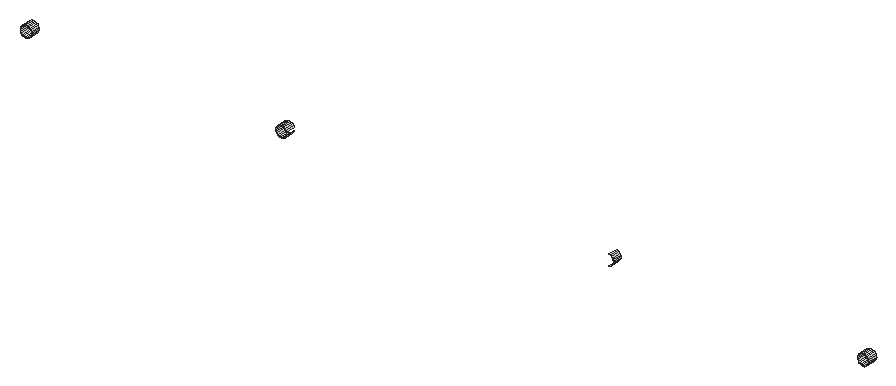
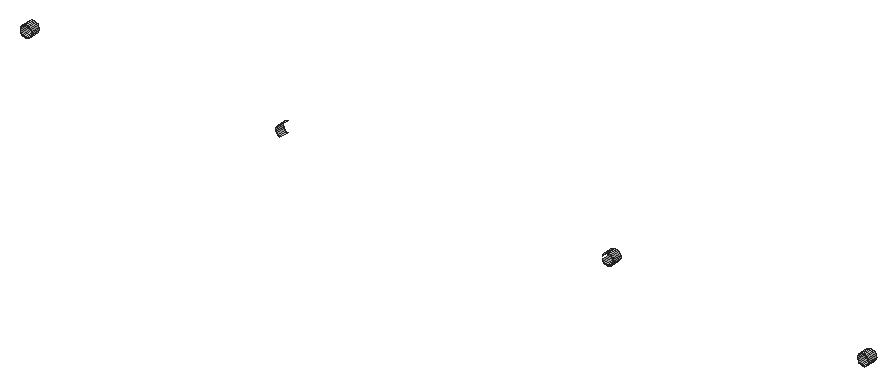
# SketchUp Ruby script. Lengths in inches.
U = 1.inch
M = Sketchup.active_model
def pt(a) = Geom::Point3d.new(a.map { |v| v * U })
def face(e, loops, mat)
  f = e.add_face(loops[0].map { |a| pt(a) })
  loops[1..].each { |l| e.add_face(l.map { |a| pt(a) }).erase! }
  f.material = f.back_material = mat if mat
  f
end
# faces: each face lists its corners as indices into pts; further lists are holes
def faces(e, pts, list, mat = nil) = list.each { |f| face(e, (f[0].is_a?(Array) ? f : [f]).map { |l| l.map { |i| pts[i] } }, mat) }
# xy, xz, yz: faces in a plane at the given z, y or x. An outline is a flat list of corners, or four numbers for a rectangle; further outlines are holes
def ring(l) = l.size == 4 ? [[l[0], l[1]], [l[2], l[1]], [l[2], l[3]], [l[0], l[3]]] : l.each_slice(2).to_a
def flat(e, list, mat, &to3) = list.each { |f| face(e, (f[0].is_a?(Array) ? f : [f]).map { |l| ring(l).map { |u, v| to3.(u, v) } }, mat) }
def xy(e, z, list, mat = nil) = flat(e, list, mat) { |x, y| [x, y, z] }
def xz(e, y, list, mat = nil) = flat(e, list, mat) { |x, z| [x, y, z] }
def yz(e, x, list, mat = nil) = flat(e, list, mat) { |y, z| [x, y, z] }
def lines(e, pts, list) = list.each { |a, b| e.add_line(pt(pts[a]), pt(pts[b])) }
# prism: a flat outline (further loops are holes) pulled along v
def prism(e, loops, v, mat = nil)
  f = face(e, loops, mat); d = Geom::Vector3d.new(v.map { |x| x * U })
  f.pushpull(f.normal.samedirection?(d) ? d.length : -d.length)
end
def box(e, o, s, mat = nil) = prism(e, [[o, [o[0] + s[0], o[1], o[2]], [o[0] + s[0], o[1] + s[1], o[2]], [o[0], o[1] + s[1], o[2]]]], [0, 0, s[2]], mat)
def at(x, y, z, deg = 0) = Geom::Transformation.translation(pt([x, y, z])) * Geom::Transformation.rotation(ORIGIN, Z_AXIS, deg.degrees)
def axes(o, x, y, z) = Geom::Transformation.new([*x, 0, *y, 0, *z, 0, *pt(o).to_a, 1])
def part(name) = M.definitions.add(name)
# library, detail: a bought-in or finely detailed component or shape, given as its bounding box
def library(name, o, s) = part(name).tap { |d| box(d.entities, o, s) }
def detail(e, o, s) = box(e.add_group.entities, o, s)
def put(e, d, t, mat = nil) = e.add_instance(d, t).tap { |i| i.material = mat if mat }
def group(e, t, mat = nil) = e.add_group.tap { |g| g.transformation = t; g.material = mat if mat }.entities
root = M.entities
p = [[2670.92,801.78,132.03],[2671.19,801.78,131.92],[2671.19,799.91,131.92],[2670.92,799.91,132.03],[2671.48,801.78,131.88],[2671.48,799.91,131.88],
  [2671.78,801.78,131.92],[2671.78,799.91,131.92],[2672.05,801.78,132.03],[2672.05,799.91,132.03],[2722.05,801.78,132.03],[2722.32,801.78,131.92],
  [2722.32,799.91,131.92],[2722.05,799.91,132.03],[2722.61,801.78,131.88],[2722.61,799.91,131.88],[2722.9,801.78,131.92],[2722.9,799.91,131.92],
  [2723.17,801.78,132.03],[2723.17,799.91,132.03],[2788.25,801.78,131.92],[2788.52,801.78,132.03],[2788.52,799.91,132.03],[2788.25,799.91,131.92],
  [2838.52,801.78,132.03],[2838.8,801.78,131.92],[2838.8,799.91,131.92],[2838.52,799.91,132.03],[2839.09,801.78,131.88],[2839.09,799.91,131.88],
  [2839.38,801.78,131.92],[2839.38,799.91,131.92],[2839.65,801.78,132.03],[2839.65,799.91,132.03],[2670.6875,801.78,132.21],[2670.6875,799.91,132.21],
  [2672.28,801.78,132.21],[2672.28,799.91,132.21],[2721.8125,801.78,132.21],[2721.8125,799.91,132.21],[2723.41,801.78,132.21],[2723.41,799.91,132.21],
  [2788.76,801.78,132.21],[2788.76,799.91,132.21],[2838.29,801.78,132.21],[2838.29,799.91,132.21],[2839.88,801.78,132.21],[2839.88,799.91,132.21],
  [2670.51,801.78,132.44],[2670.51,799.91,132.44],[2672.46,801.78,132.44],[2672.46,799.91,132.44],[2721.64,801.78,132.44],[2721.64,799.91,132.44],
  [2723.58,801.78,132.44],[2723.58,799.91,132.44],[2788.94,801.78,132.44],[2788.94,799.91,132.44],[2838.11,801.78,132.44],[2838.11,799.91,132.44],
  [2840.06,801.78,132.44],[2840.06,799.91,132.44],[2670.4,801.78,132.71],[2670.4,799.91,132.71],[2672.57,801.78,132.71],[2672.57,799.91,132.71],
  [2721.52,801.78,132.71],[2721.52,799.91,132.71],[2723.7,801.78,132.71],[2723.7,799.91,132.71],[2789.05,801.78,132.71],[2789.05,799.91,132.71],
  [2838,801.78,132.71],[2838,799.91,132.71],[2840.17,801.78,132.71],[2840.17,799.91,132.71],[2670.36,801.78,133],[2670.36,799.91,133],
  [2672.61,801.78,133],[2672.61,799.91,133],[2721.48,801.78,133],[2721.48,799.91,133],[2789.09,801.78,133],[2789.09,799.91,133],
  [2837.96,801.78,133],[2837.96,799.91,133],[2840.21,801.78,133],[2840.21,799.91,133],[2670.4,801.78,133.29],[2670.4,799.91,133.29],
  [2672.57,801.78,133.29],[2672.57,799.91,133.29],[2721.52,801.78,133.29],[2721.52,799.91,133.29],[2789.05,801.78,133.29],[2789.05,799.91,133.29],
  [2838,801.78,133.29],[2838,799.91,133.29],[2840.17,801.78,133.29],[2840.17,799.91,133.29],[2670.51,801.78,133.57],[2670.51,799.91,133.57],
  [2672.46,801.78,133.57],[2672.46,799.91,133.57],[2721.64,801.78,133.57],[2721.64,799.91,133.57],[2723.7,801.78,133.29],[2723.58,801.78,133.57],
  [2723.58,799.91,133.57],[2723.7,799.91,133.29],[2788.94,801.78,133.57],[2788.94,799.91,133.57],[2838.11,801.78,133.57],[2838.11,799.91,133.57],
  [2840.06,801.78,133.57],[2840.06,799.91,133.57],[2670.6875,801.78,133.8],[2670.6875,799.91,133.8],[2672.28,801.78,133.8],[2672.28,799.91,133.8],
  [2721.8125,801.78,133.8],[2721.8125,799.91,133.8],[2723.41,801.78,133.8],[2723.41,799.91,133.8],[2788.76,801.78,133.8],[2788.76,799.91,133.8],
  [2838.29,801.78,133.8],[2838.29,799.91,133.8],[2839.88,801.78,133.8],[2839.88,799.91,133.8],[2670.92,801.78,133.98],[2670.92,799.91,133.98],
  [2672.05,801.78,133.98],[2672.05,799.91,133.98],[2722.05,801.78,133.98],[2722.05,799.91,133.98],[2723.17,801.78,133.98],[2723.17,799.91,133.98],
  [2788.52,801.78,133.98],[2788.52,799.91,133.98],[2838.52,801.78,133.98],[2838.52,799.91,133.98],[2839.65,801.78,133.98],[2839.65,799.91,133.98],
  [2671.19,801.78,134.09],[2671.19,799.91,134.09],[2671.78,801.78,134.09],[2671.78,799.91,134.09],[2722.32,801.78,134.09],[2722.32,799.91,134.09],
  [2722.9,801.78,134.09],[2722.9,799.91,134.09],[2788.25,801.78,134.09],[2788.25,799.91,134.09],[2838.8,801.78,134.09],[2838.8,799.91,134.09],
  [2839.38,801.78,134.09],[2839.38,799.91,134.09],[2671.48,801.78,134.13],[2671.48,799.91,134.13],[2722.61,801.78,134.13],[2722.61,799.91,134.13],
  [2839.09,801.78,134.13],[2839.09,799.91,134.13]]
faces(root,p,[[0,1,2,3],[1,4,5,2],[4,6,7,5],[6,8,9,7],[10,11,12,13],[11,14,15,12],[14,16,17,15],[16,18,19,17],
  [20,21,22,23],[24,25,26,27],[25,28,29,26],[28,30,31,29],[30,32,33,31],[34,0,3,35],[8,36,37,9],[38,10,13,39],
  [18,40,41,19],[21,42,43,22],[44,24,27,45],[32,46,47,33],[48,34,35,49],[36,50,51,37],[52,38,39,53],[40,54,55,41],
  [42,56,57,43],[58,44,45,59],[46,60,61,47],[62,48,49,63],[50,64,65,51],[66,52,53,67],[54,68,69,55],[56,70,71,57],
  [72,58,59,73],[60,74,75,61],[76,62,63,77],[64,78,79,65],[80,66,67,81],[70,82,83,71],[84,72,73,85],[74,86,87,75],
  [88,76,77,89],[78,90,91,79],[92,80,81,93],[82,94,95,83],[96,84,85,97],[86,98,99,87],[100,88,89,101],[90,102,103,91],
  [104,92,93,105],[106,107,108,109],[94,110,111,95],[112,96,97,113],[98,114,115,99],[116,100,101,117],[102,118,119,103],[120,104,105,121],
  [107,122,123,108],[110,124,125,111],[126,112,113,127],[114,128,129,115],[130,116,117,131],[118,132,133,119],[134,120,121,135],[122,136,137,123],
  [124,138,139,125],[140,126,127,141],[128,142,143,129],[144,130,131,145],[132,146,147,133],[148,134,135,149],[136,150,151,137],[138,152,153,139],
  [154,140,141,155],[142,156,157,143],[158,144,145,159],[146,158,159,147],[160,148,149,161],[150,160,161,151],[162,154,155,163],[156,162,163,157]])
